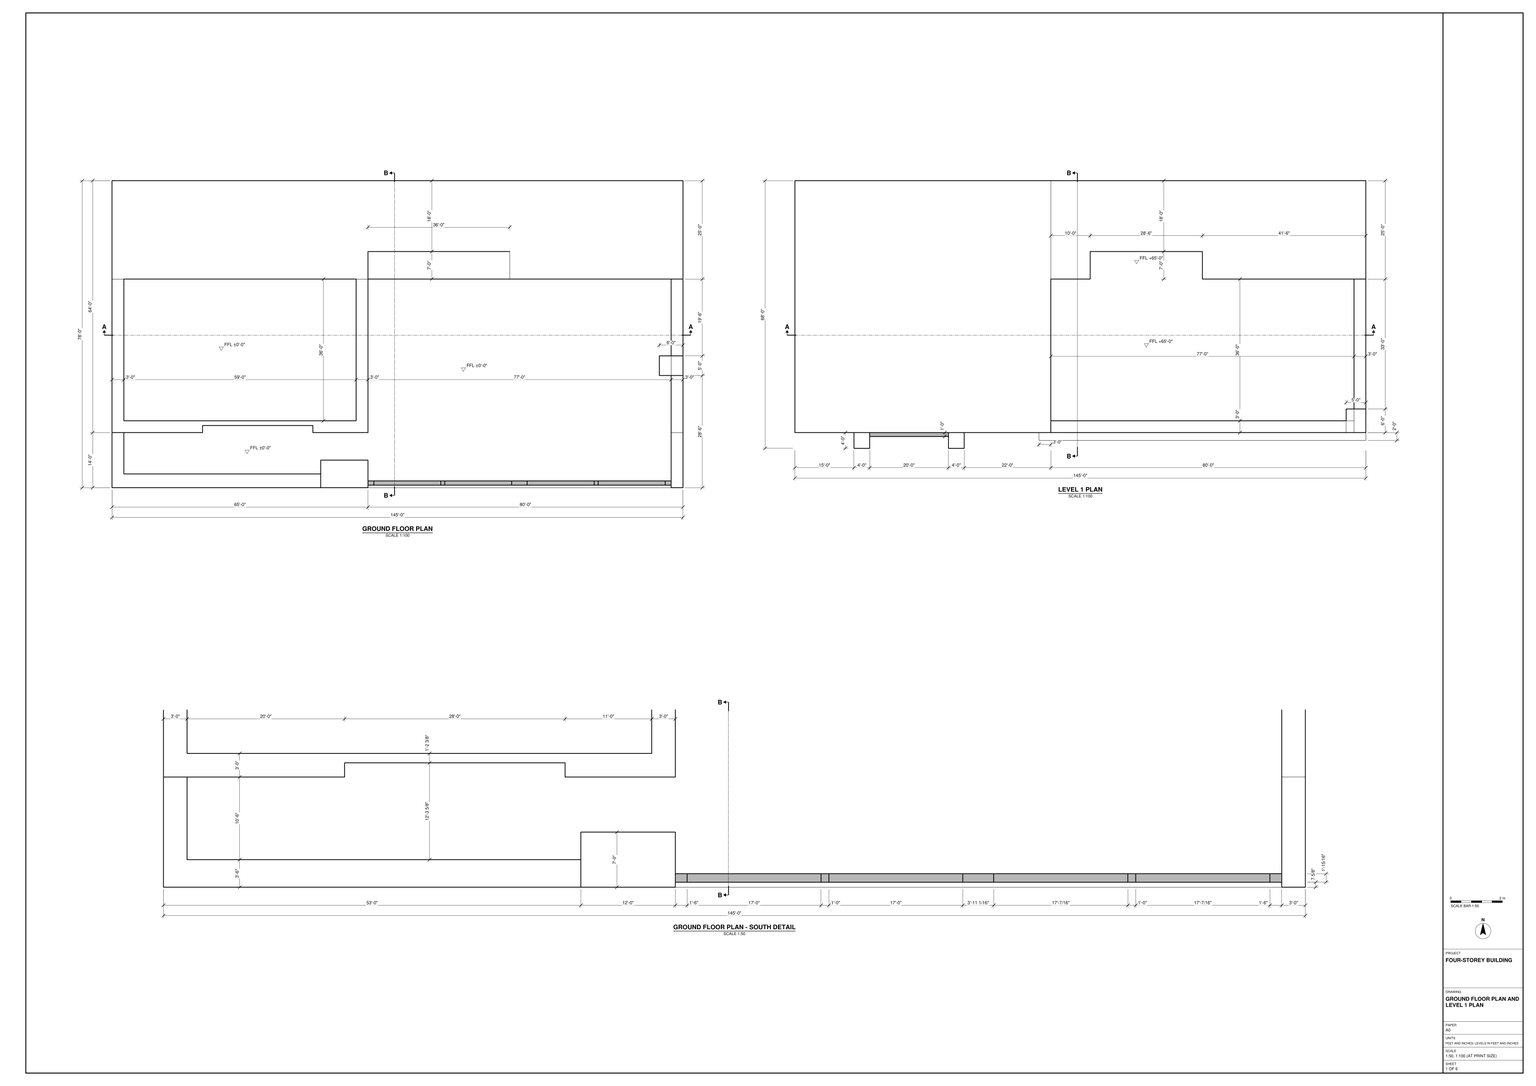
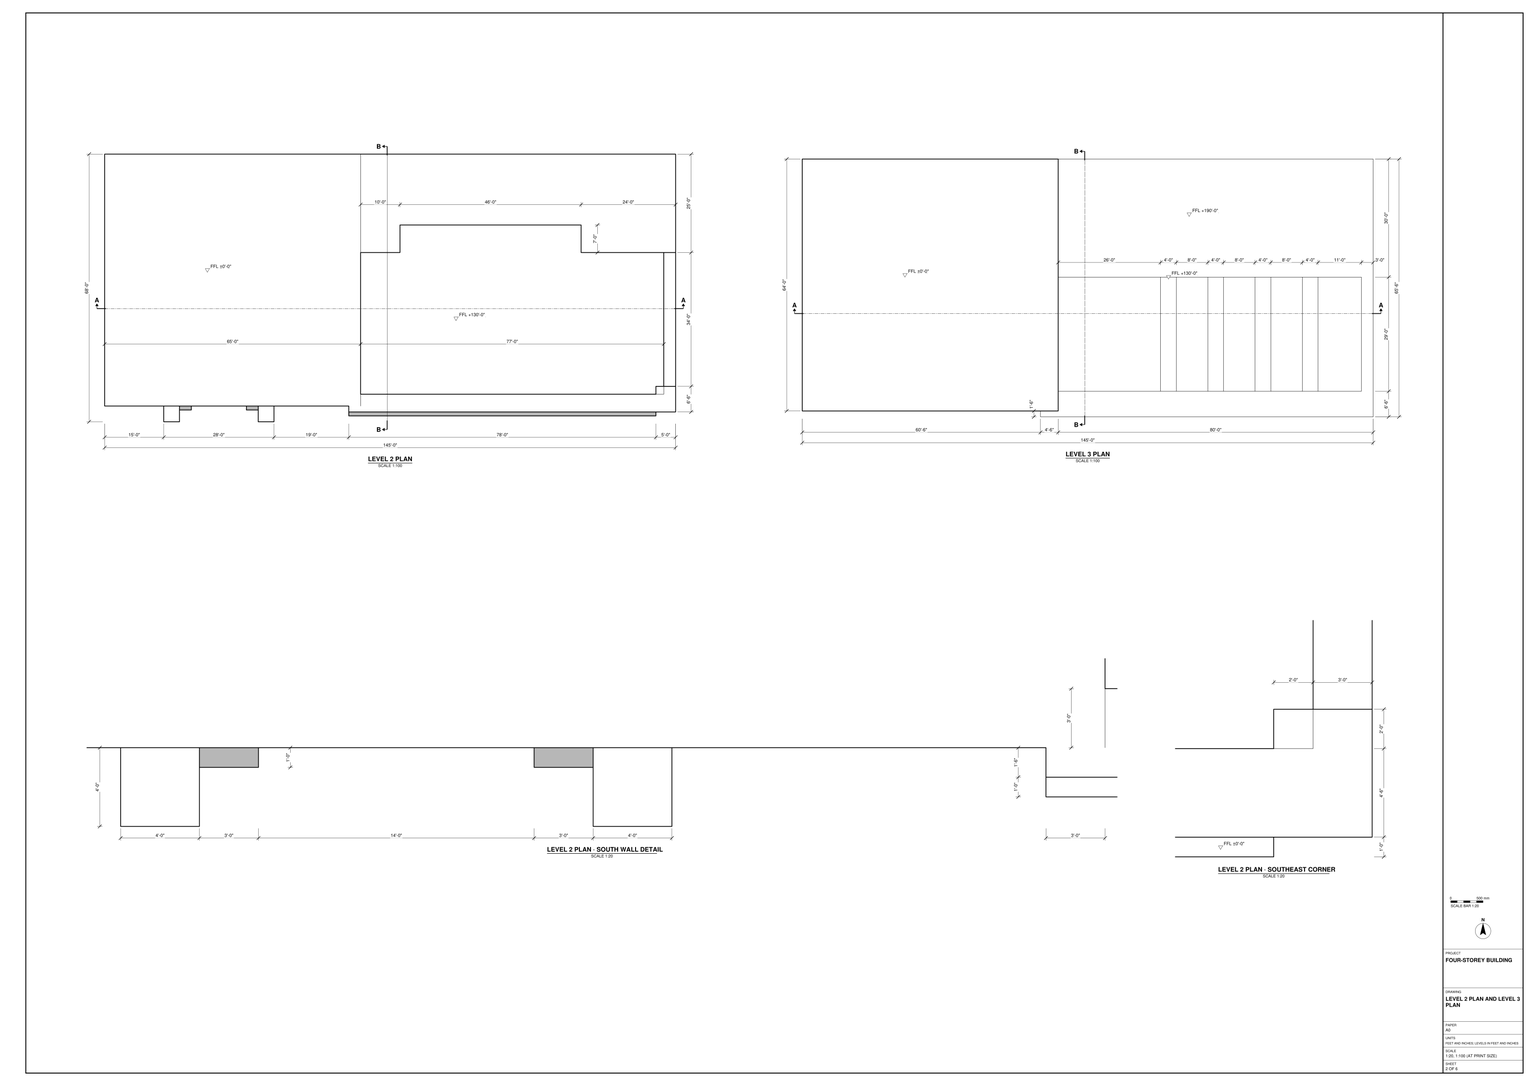
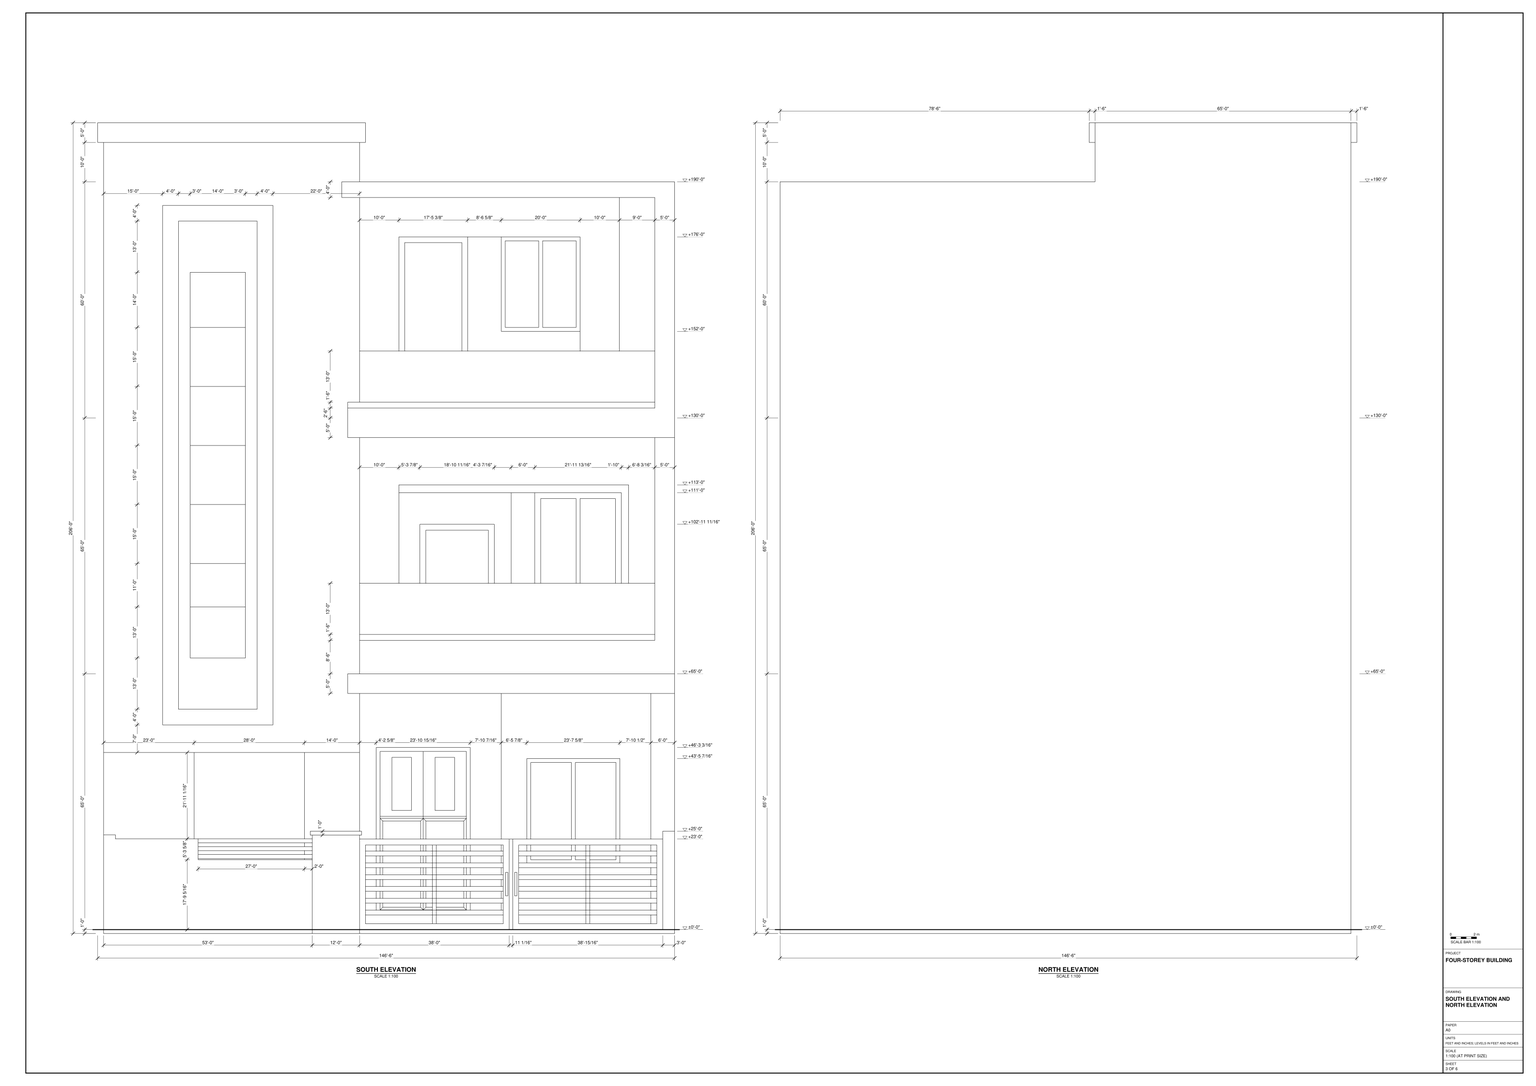
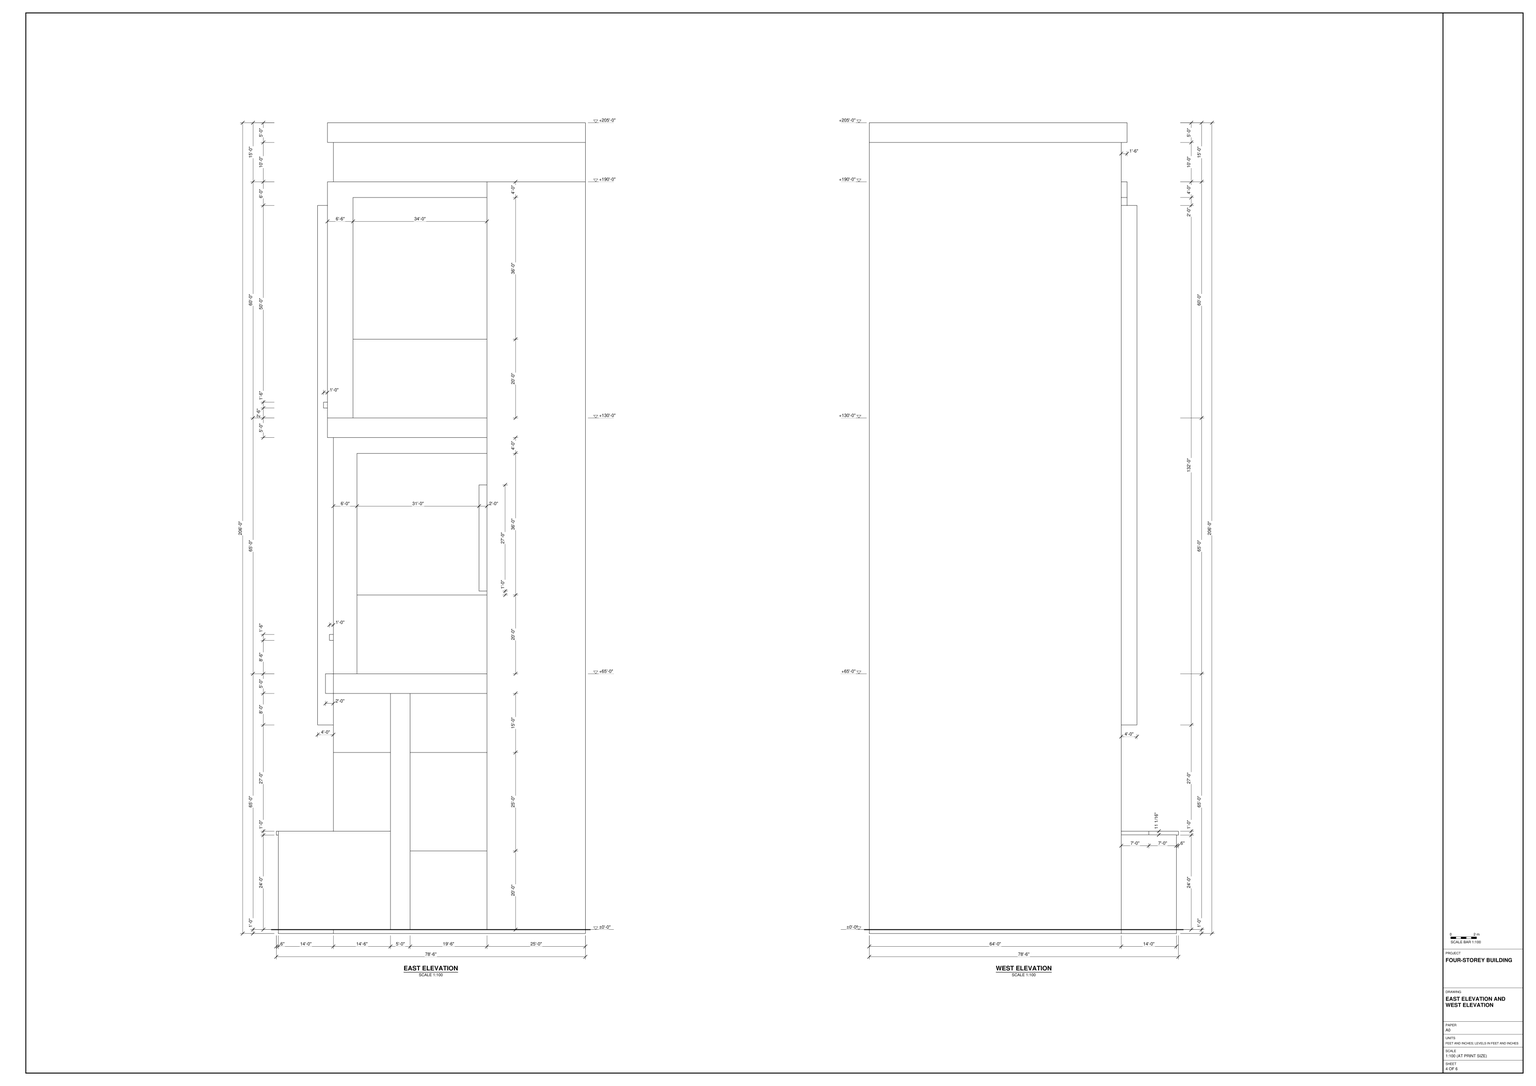
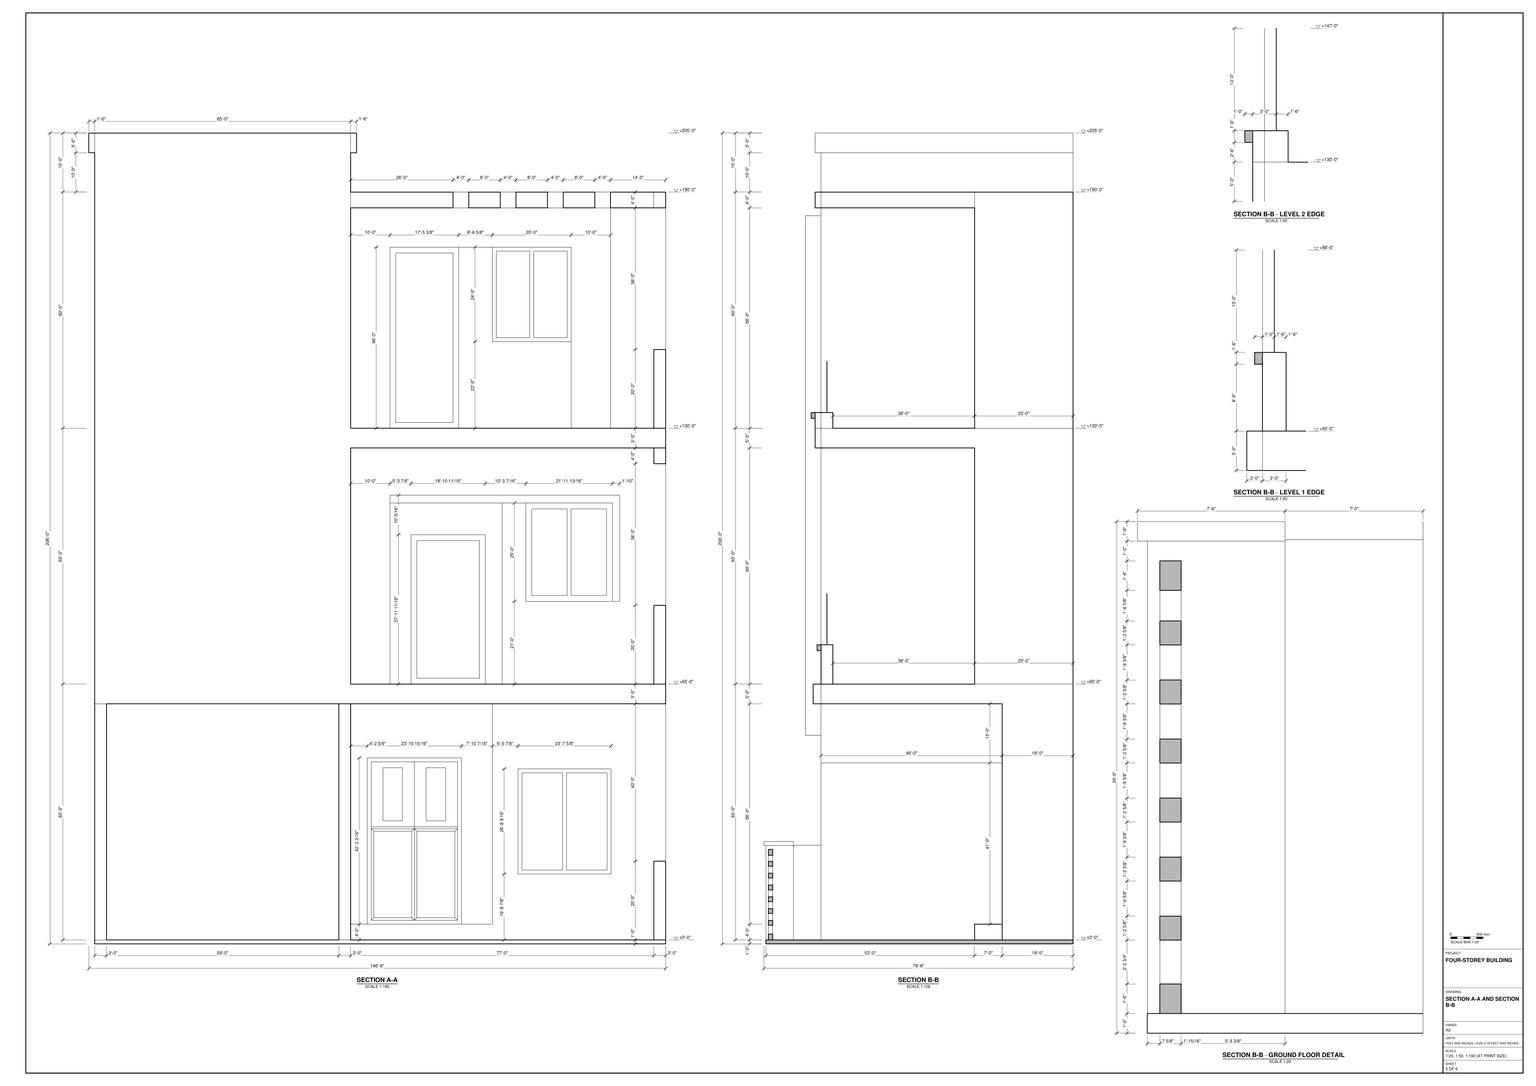
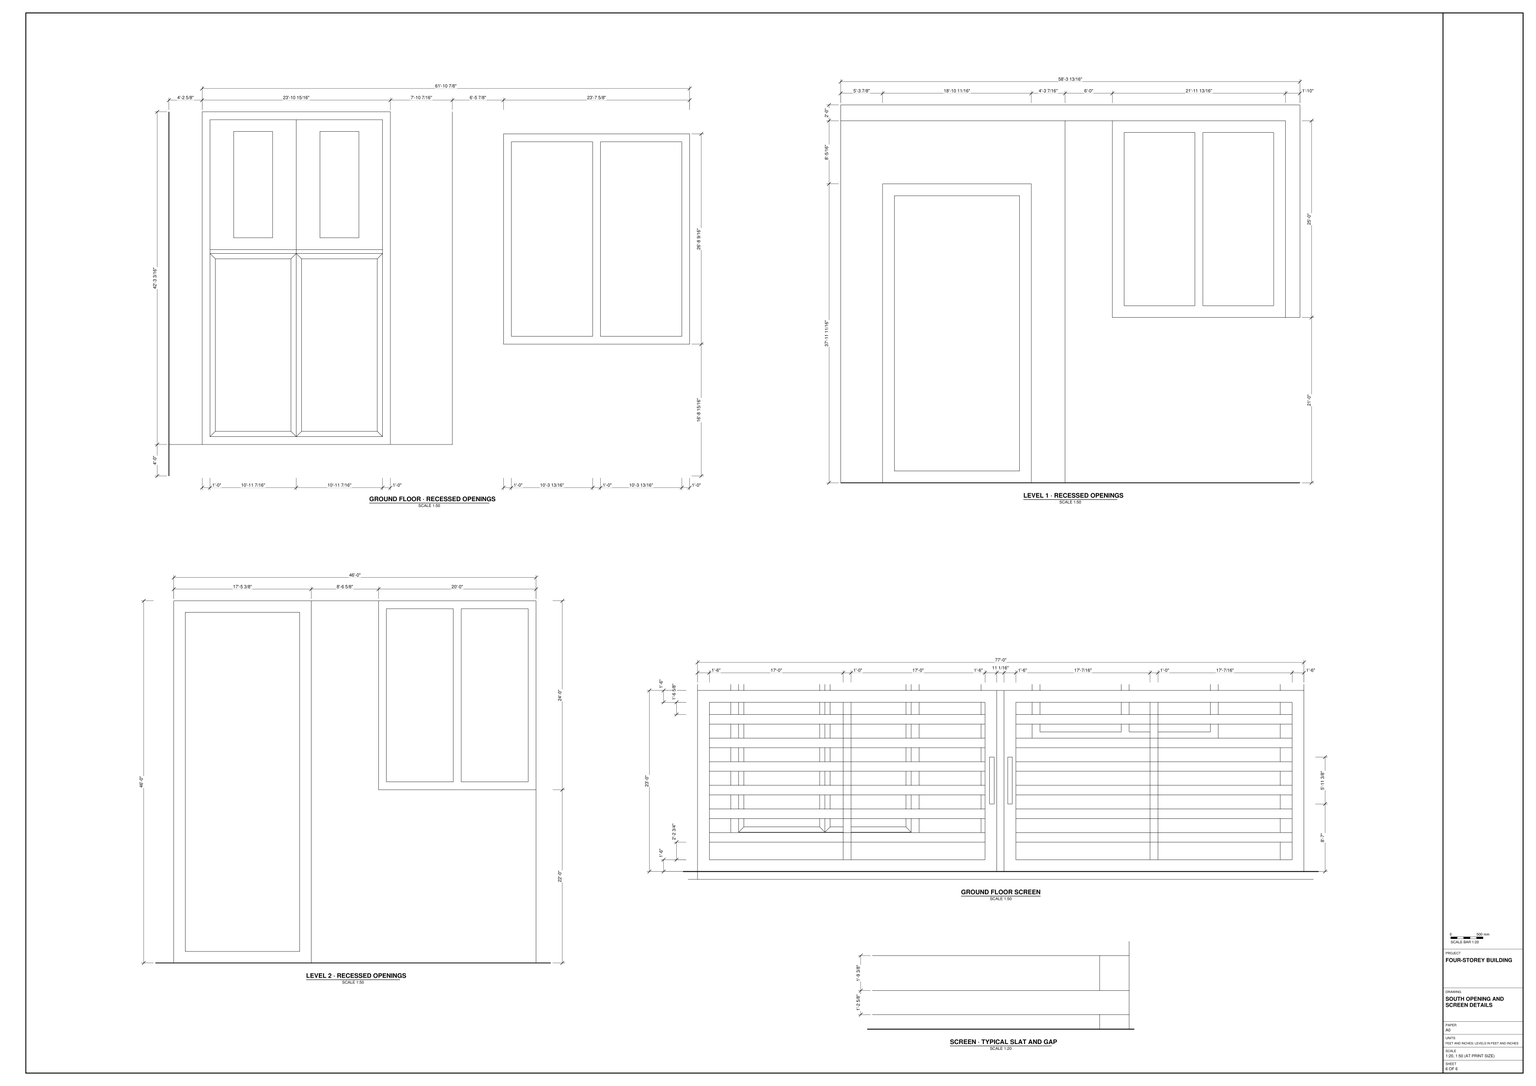
Build the four-storey building in SketchUp from task_files/diagram_01.pdf. Work in feet and inches, with the south frontage along the x-axis and the building depth along the y-axis. Including projections, the overall model shall be 146'-6" wide, 78'-6" deep and 206'-0" high. Set the floor levels at ±0'-0", +65'-0", +130'-0" and +190'-0" relative to the ground floor.

Use the plans to trace the wall returns at their drawn thicknesses and to shape the slabs and roof at each level. On the south elevation, distinguish the taller western block, with its projecting roof cap and tall framed panel, from the eastern bays. Set the upper doors and windows behind the balcony fronts so the recesses have depth. At ground level, model the frontage wall, piers and horizontally slatted gates in front of the openings. Follow the level 3 plan for the arrangement of parallel members over the eastern bays, and retain the plain stepped profile on the north elevation.

Keep shell elements such as walls, slabs and roof in separate groups or components. Keep each furniture or joinery piece shown separate as well, and use components for repeated parts. Any decor or loose items shown may use suitable library components. Save one SketchUp model as output_files/four_storey_building_with_recessed_south_balconies.skp.

# SketchUp Ruby script. Lengths in inches.
U = 1.inch
M = Sketchup.active_model
def pt(a) = Geom::Point3d.new(a.map { |v| v * U })
def face(e, loops, mat)
  f = e.add_face(loops[0].map { |a| pt(a) })
  loops[1..].each { |l| e.add_face(l.map { |a| pt(a) }).erase! }
  f.material = f.back_material = mat if mat
  f
end
# faces: each face lists its corners as indices into pts; further lists are holes
def faces(e, pts, list, mat = nil) = list.each { |f| face(e, (f[0].is_a?(Array) ? f : [f]).map { |l| l.map { |i| pts[i] } }, mat) }
# xy, xz, yz: faces in a plane at the given z, y or x. An outline is a flat list of corners, or four numbers for a rectangle; further outlines are holes
def ring(l) = l.size == 4 ? [[l[0], l[1]], [l[2], l[1]], [l[2], l[3]], [l[0], l[3]]] : l.each_slice(2).to_a
def flat(e, list, mat, &to3) = list.each { |f| face(e, (f[0].is_a?(Array) ? f : [f]).map { |l| ring(l).map { |u, v| to3.(u, v) } }, mat) }
def xy(e, z, list, mat = nil) = flat(e, list, mat) { |x, y| [x, y, z] }
def xz(e, y, list, mat = nil) = flat(e, list, mat) { |x, z| [x, y, z] }
def yz(e, x, list, mat = nil) = flat(e, list, mat) { |y, z| [x, y, z] }
def lines(e, pts, list) = list.each { |a, b| e.add_line(pt(pts[a]), pt(pts[b])) }
# prism: a flat outline (further loops are holes) pulled along v
def prism(e, loops, v, mat = nil)
  f = face(e, loops, mat); d = Geom::Vector3d.new(v.map { |x| x * U })
  f.pushpull(f.normal.samedirection?(d) ? d.length : -d.length)
end
def box(e, o, s, mat = nil) = prism(e, [[o, [o[0] + s[0], o[1], o[2]], [o[0] + s[0], o[1] + s[1], o[2]], [o[0], o[1] + s[1], o[2]]]], [0, 0, s[2]], mat)
def at(x, y, z, deg = 0) = Geom::Transformation.translation(pt([x, y, z])) * Geom::Transformation.rotation(ORIGIN, Z_AXIS, deg.degrees)
def axes(o, x, y, z) = Geom::Transformation.new([*x, 0, *y, 0, *z, 0, *pt(o).to_a, 1])
def part(name) = M.definitions.add(name)
# library, detail: a bought-in or finely detailed component or shape, given as its bounding box
def library(name, o, s) = part(name).tap { |d| box(d.entities, o, s) }
def detail(e, o, s) = box(e.add_group.entities, o, s)
def put(e, d, t, mat = nil) = e.add_instance(d, t).tap { |i| i.material = mat if mat }
def group(e, t, mat = nil) = e.add_group.tap { |g| g.transformation = t; g.material = mat if mat }.entities
root = M.entities
M.materials.add("[0022_Maroon]").color = [71, 0, 0]
M.materials.add("[0033_NavajoWhite]").color = [255, 222, 173]
M.materials.add("[0057_DarkKhaki]").color = [189, 183, 107]
M.materials.add("[0060_GrassGreen]").color = [62, 91, 5]
M.materials.add("[0061_OliveDrab]").color = [113, 150, 37]
M.materials.add("[Cladding Siding White]").color = [168, 161, 129]
M.materials.add("[Granite Dark Gray]").color = [69, 68, 68]
M.materials.add("[Stone Marble]").color = [143, 138, 136]
M.materials.add("[Translucent Glass Gray]").color = [204, 221, 91]
M.materials["[Translucent Glass Gray]"].alpha = 0.5
M.materials.add("[Translucent Glass Gray]1").color = [128, 128, 128]
M.materials["[Translucent Glass Gray]1"].alpha = 0.5
M.materials.add("[Wood Bamboo]").color = [150, 89, 36]
M.materials.add("[Wood Cherry Original]").color = [152, 86, 42]
M.materials.add("[Wood Veneer 01]").color = [120, 70, 37]
xy(root,0,[[18,6,18,174,294,174,294,195.6,630,195.6,630,6],[630,6,1758,174],[18,174,18,942,1758,942,1758,174,630,174,630,195.6,294,195.6,294,174]])
xy(root,12,[[18,6,18,174,54,174,54,48,654,48,654,6],[798,6,1722,13.64],[1722,6,1758,174],[798,13.64,1722,26.59],[1722,174,1758,348],
  [54,210,762,642],[1686,348,1722,408],[1722,348,1758,408],[1722,408,1758,642],[18,642,18,942,1758,942,1758,642,1230,642,1230,726,798,726,798,642],
  [798,642,1230,726]])
xy(root,12,[[798,26.59,1722,26.59,1722,348,1686,348,1686,408,1722,408,1722,642,798,642,798,174,630,174,630,195.6,294,195.6,294,174,54,174,54,48,654,48,654,90,798,90]],"[Granite Dark Gray]")
xy(root,30,[[816,13.64,1020,26.59],[1032,13.64,1236,26.59],[1283.08,13.64,1487.54,26.59],[1499.54,13.64,1704,26.59]])
xy(root,56.76,[[816,13.64,1236,26.59],[1283.08,13.64,1704,26.59]])
xy(root,60,[[798,642,1230,726]],"[0057_DarkKhaki]")
xy(root,71.36,[[816,13.64,1236,26.59],[1283.08,13.64,1704,26.59]])
xy(root,92.76,[[816,13.64,1236,26.59],[1283.08,13.64,1704,26.59]])
xy(root,107.36,[[816,13.64,1236,26.59],[1283.08,13.64,1704,26.59]])
xy(root,128.76,[[816,13.64,1236,26.59],[1283.08,13.64,1704,26.59]])
xy(root,143.36,[[816,13.64,1236,26.59],[1283.08,13.64,1704,26.59]])
xy(root,164.76,[[816,13.64,1236,26.59],[1283.08,13.64,1704,26.59]])
xy(root,179.36,[[816,13.64,1236,26.59],[1283.08,13.64,1704,26.59]])
xy(root,200.76,[[816,13.64,1236,26.59],[1283.08,13.64,1704,26.59]])
xy(root,215.36,[[816,13.64,1236,26.59],[1283.08,13.64,1704,26.59]])
xy(root,225.34,[[306,6,654,48]],"[0033_NavajoWhite]")
xy(root,228.5,[[306,16.5,654,38.4375]])
xy(root,236.76,[[816,13.64,1236,26.59],[1283.08,13.64,1704,26.59]])
xy(root,240.9375,[[306,16.5,654,38.4375]])
xy(root,251.36,[[816,13.64,1236,26.59],[1283.08,13.64,1704,26.59]])
xy(root,252,[[1722,408,1758,642]],"[0033_NavajoWhite]")
xy(root,252.5,[[306,16.5,654,38.4375]])
xy(root,264.9375,[[306,16.5,654,38.4375]])
xy(root,270,[[816,13.64,1020,26.59],[1032,13.64,1236,26.59],[1283.08,13.64,1487.54,26.59],[1499.54,13.64,1704,26.59]])
xy(root,276.5,[[306,16.5,654,38.4375]])
xy(root,288,[[798,13.64,1722,26.59]])
xy(root,288.9375,[[306,16.5,654,38.4375]])
xy(root,288.9375,[[54,6,306,48]],"[0033_NavajoWhite]")
xy(root,300,[[648,0,654,6],[654,0,654,6,798,6,798,90,804,90,804,0],[648,6,654,90]])
xy(root,300.9375,[[18,6,54,174]],"[0033_NavajoWhite]")
xy(root,312,[[648,0,804,90]])
xy(root,312,[[1722,6,1758,348]],"[0033_NavajoWhite]")
xy(root,552,[[294,174,630,195.6]],"[0061_OliveDrab]")
xy(root,636,[[198,126,534,174]])
xy(root,684,[[246,126,486,162],[246,162,486,174]])
xy(root,732,[[762,174,798,642],[54,210,762,642],[862.31,212.47,857.66,213.09,853.31,214.89,849.59,217.75,846.73,221.47,844.93,225.82,844.31,230.47,844.93,235.13,846.73,239.47,849.59,243.2,853.31,246.0625,857.66,247.86,862.31,248.47,866.97,247.86,871.31,246.0625,875.04,243.2,877.9,239.47,879.7,235.13,880.31,230.47,879.7,225.82,877.9,221.47,875.04,217.75,871.31,214.89,866.97,213.09],[1042.31,212.47,1037.66,213.09,1033.31,214.89,1029.59,217.75,1026.73,221.47,1024.93,225.82,1024.31,230.47,1024.93,235.13,1026.73,239.47,1029.59,243.2,1033.31,246.0625,1037.66,247.86,1042.31,248.47,1046.97,247.86,1051.31,246.0625,1055.04,243.2,1057.9,239.47,1059.7,235.13,1060.31,230.47,1059.7,225.82,1057.9,221.47,1055.04,217.75,1051.31,214.89,1046.97,213.09],[1222.31,212.47,1217.66,213.09,1213.31,214.89,1209.59,217.75,1206.73,221.47,1204.93,225.82,1204.31,230.47,1204.93,235.13,1206.73,239.47,1209.59,243.2,1213.31,246.0625,1217.66,247.86,1222.31,248.47,1226.97,247.86,1231.31,246.0625,1235.04,243.2,1237.9,239.47,1239.7,235.13,1240.31,230.47,1239.7,225.82,1237.9,221.47,1235.04,217.75,1231.31,214.89,1226.97,213.09],
  [1402.31,212.47,1397.66,213.09,1393.31,214.89,1389.59,217.75,1386.73,221.47,1384.93,225.82,1384.31,230.47,1384.93,235.13,1386.73,239.47,1389.59,243.2,1393.31,246.0625,1397.66,247.86,1402.31,248.47,1406.97,247.86,1411.31,246.0625,1415.04,243.2,1417.9,239.47,1419.7,235.13,1420.31,230.47,1419.7,225.82,1417.9,221.47,1415.04,217.75,1411.31,214.89,1406.97,213.09],[1582.31,212.47,1577.66,213.09,1573.31,214.89,1569.59,217.75,1566.73,221.47,1564.93,225.82,1564.31,230.47,1564.93,235.13,1566.73,239.47,1569.59,243.2,1573.31,246.0625,1577.66,247.86,1582.31,248.47,1586.97,247.86,1591.31,246.0625,1595.04,243.2,1597.9,239.47,1599.7,235.13,1600.31,230.47,1599.7,225.82,1597.9,221.47,1595.04,217.75,1591.31,214.89,1586.97,213.09],[1686,348,1758,408]])
xy(root,732,[[[762,150,762,174,798,174,798,726,1230,726,1230,642,1758,642,1758,408,1686,408,1686,348,1758,348,1758,150],[862.31,212.47,866.97,213.09,871.31,214.89,875.04,217.75,877.9,221.47,879.7,225.82,880.31,230.47,879.7,235.13,877.9,239.47,875.04,243.2,871.31,246.0625,866.97,247.86,862.31,248.47,857.66,247.86,853.31,246.0625,849.59,243.2,846.73,239.47,844.93,235.13,844.31,230.47,844.93,225.82,846.73,221.47,849.59,217.75,853.31,214.89,857.66,213.09],[1042.31,212.47,1046.97,213.09,1051.31,214.89,1055.04,217.75,1057.9,221.47,1059.7,225.82,1060.31,230.47,1059.7,235.13,1057.9,239.47,1055.04,243.2,1051.31,246.0625,1046.97,247.86,1042.31,248.47,1037.66,247.86,1033.31,246.0625,1029.59,243.2,1026.73,239.47,1024.93,235.13,1024.31,230.47,1024.93,225.82,1026.73,221.47,1029.59,217.75,1033.31,214.89,1037.66,213.09],[1222.31,212.47,1226.97,213.09,1231.31,214.89,1235.04,217.75,1237.9,221.47,1239.7,225.82,1240.31,230.47,1239.7,235.13,1237.9,239.47,1235.04,243.2,1231.31,246.0625,1226.97,247.86,1222.31,248.47,1217.66,247.86,1213.31,246.0625,1209.59,243.2,1206.73,239.47,1204.93,235.13,1204.31,230.47,1204.93,225.82,1206.73,221.47,1209.59,217.75,1213.31,214.89,1217.66,213.09],[1402.31,212.47,1406.97,213.09,1411.31,214.89,1415.04,217.75,1417.9,221.47,1419.7,225.82,1420.31,230.47,1419.7,235.13,1417.9,239.47,1415.04,243.2,1411.31,246.0625,1406.97,247.86,1402.31,248.47,1397.66,247.86,1393.31,246.0625,1389.59,243.2,1386.73,239.47,1384.93,235.13,1384.31,230.47,1384.93,225.82,1386.73,221.47,1389.59,217.75,1393.31,214.89,1397.66,213.09],[1582.31,212.47,1586.97,213.09,1591.31,214.89,1595.04,217.75,1597.9,221.47,1599.7,225.82,1600.31,230.47,1599.7,235.13,1597.9,239.47,1595.04,243.2,1591.31,246.0625,1586.97,247.86,1582.31,248.47,1577.66,247.86,1573.31,246.0625,1569.59,243.2,1566.73,239.47,1564.93,235.13,1564.31,230.47,1564.93,225.82,1566.73,221.47,1569.59,217.75,1573.31,214.89,1577.66,213.09]]],"[Wood Cherry Original]")
xy(root,792,[[798,174,1698,210],[1698,174,1722,210],[1722,174,1758,246],[1698,210,1722,246],[1722,246,1758,642]])
xy(root,792,[[762,150,1758,174]],"[0060_GrassGreen]")
xy(root,792,[[798,210,1698,210,1698,246,1722,246,1722,642,1260,642,1260,726,918,726,918,642,798,642]],"[Stone Marble]")
xy(root,840,[[282,162,450,174]])
xy(root,894,[[798,162,1698,174]])
xy(root,912,[[798,162,1698,174],[798,174,1698,192],[798,192,1698,210]])
xy(root,1032,[[1722,246,1758,642]],"[0033_NavajoWhite]")
xy(root,1044,[[1595.8125,618,1617.8125,642]])
xy(root,1344,[[918,618,918,726,1260,726,1260,642,1595.8125,642,1595.8125,618]],"[Wood Bamboo]")
xy(root,1368,[[918,618,1617.8125,642]])
xy(root,1464,[[1722,246,1758,642]])
xy(root,1512,[[1698,174,1722,246],[1722,174,1758,642],[964.25,258.46,958.07,259.49,952.37,262.08,947.53,266.06,943.89,271.16,941.6875,277.02,941.08,283.26,942.11,289.44,944.7,295.14,948.68,299.98,953.78,303.625,959.65,305.82,965.88,306.43,972.0625,305.4,977.77,302.8125,982.6,298.83,986.25,293.73,988.45,287.87,989.05,281.63,988.03,275.45,985.43,269.75,981.45,264.91,976.36,261.27,970.49,259.07],[1228.25,258.46,1222.07,259.49,1216.37,262.08,1211.53,266.06,1207.89,271.16,1205.6875,277.02,1205.08,283.26,1206.11,289.44,1208.7,295.14,1212.68,299.98,1217.78,303.625,1223.65,305.82,1229.88,306.43,1236.0625,305.4,1241.77,302.8125,1246.6,298.83,1250.25,293.73,1252.45,287.87,1253.05,281.63,1252.03,275.45,1249.43,269.75,1245.45,264.91,1240.36,261.27,1234.49,259.07],[1492.25,258.46,1486.07,259.49,1480.37,262.08,1475.53,266.06,1471.89,271.16,1469.6875,277.02,1469.08,283.26,1470.11,289.44,1472.7,295.14,1476.68,299.98,1481.78,303.625,1487.65,305.82,1493.88,306.43,1500.0625,305.4,1505.77,302.8125,1510.6,298.83,1514.25,293.73,1516.45,287.87,1517.05,281.63,1516.03,275.45,1513.43,269.75,1509.45,264.91,1504.36,261.27,1498.49,259.07]])
xy(root,1512,[[[762,156,762,174,798,174,798,642,1722,642,1722,246,1698,246,1698,174,1758,174,1758,156],[1228.25,258.46,1234.49,259.07,1240.36,261.27,1245.45,264.91,1249.43,269.75,1252.03,275.45,1253.05,281.63,1252.45,287.87,1250.25,293.73,1246.6,298.83,1241.77,302.8125,1236.0625,305.4,1229.88,306.43,1223.65,305.82,1217.78,303.625,1212.68,299.98,1208.7,295.14,1206.11,289.44,1205.08,283.26,1205.6875,277.02,1207.89,271.16,1211.53,266.06,1216.37,262.08,1222.07,259.49],[1492.25,258.46,1498.49,259.07,1504.36,261.27,1509.45,264.91,1513.43,269.75,1516.03,275.45,1517.05,281.63,1516.45,287.87,1514.25,293.73,1510.6,298.83,1505.77,302.8125,1500.0625,305.4,1493.88,306.43,1487.65,305.82,1481.78,303.625,1476.68,299.98,1472.7,295.14,1470.11,289.44,1469.08,283.26,1469.6875,277.02,1471.89,271.16,1475.53,266.06,1480.37,262.08,1486.07,259.49],[964.25,258.46,970.49,259.07,976.36,261.27,981.45,264.91,985.43,269.75,988.03,275.45,989.05,281.63,988.45,287.87,986.25,293.73,982.6,298.83,977.77,302.8125,972.0625,305.4,965.88,306.43,959.65,305.82,953.78,303.625,948.68,299.98,944.7,295.14,942.11,289.44,941.08,283.26,941.6875,277.02,943.89,271.16,947.53,266.06,952.37,262.08,958.07,259.49]]],"[Wood Cherry Original]")
xy(root,1572,[[1698,210,1722,234],[1722,234,1758,642]])
xy(root,1572,[[798,210,1698,210,1698,234,1722,234,1722,642,1470,642,1470,726,918,726,918,642,798,642]],"[Stone Marble]")
xy(root,1602,[[762,144,1698,156]])
xy(root,1620,[[762,144,1698,156],[762,156,1698,156,1698,192,798,192,798,174,762,174],[798,192,1698,210]])
xy(root,1812,[[1722,234,1758,642]],"[0033_NavajoWhite]")
xy(root,2016,[[282,162,450,174]])
xy(root,2124,[[918,642,1127.375,726],[1127.375,642,1470,726]],"[Wood Bamboo]")
xy(root,2172,[[246,126,486,162],[246,162,486,174]])
xy(root,2220,[[198,126,534,174]])
xy(root,2244,[[978.39,287.6,973.73,288.22,969.39,290.02,965.66,292.875,962.8,296.6,961,300.95,960.39,305.6,961,310.26,962.8,314.6,965.66,318.33,969.39,321.19,973.73,322.99,978.39,323.6,983.04,322.99,987.39,321.19,991.11,318.33,993.97,314.6,995.77,310.26,996.39,305.6,995.77,300.95,993.97,296.6,991.11,292.875,987.39,290.02,983.04,288.22],[1660.26,287.6,1655.6,288.22,1651.26,290.02,1647.53,292.875,1644.67,296.6,1642.875,300.95,1642.26,305.6,1642.875,310.26,1644.67,314.6,1647.53,318.33,1651.26,321.19,1655.6,322.99,1660.26,323.6,1664.92,322.99,1669.26,321.19,1672.99,318.33,1675.85,314.6,1677.65,310.26,1678.26,305.6,1677.65,300.95,1675.85,296.6,1672.99,292.875,1669.26,290.02,1664.92,288.22],[978.39,442.12,973.73,442.73,969.39,444.53,965.66,447.39,962.8,451.12,961,455.46,960.39,460.12,961,464.78,962.8,469.12,965.66,472.85,969.39,475.71,973.73,477.51,978.39,478.12,983.04,477.51,987.39,475.71,991.11,472.85,993.97,469.12,995.77,464.78,996.39,460.12,995.77,455.46,993.97,451.12,991.11,447.39,987.39,444.53,983.04,442.73],[1660.26,443.92,1655.6,444.53,1651.26,446.33,1647.53,449.1875,1644.67,452.92,1642.875,457.26,1642.26,461.92,1642.875,466.58,1644.67,470.92,1647.53,474.65,1651.26,477.51,1655.6,479.3,1660.26,479.92,1664.92,479.3,1669.26,477.51,1672.99,474.65,1675.85,470.92,1677.65,466.58,1678.26,461.92,1677.65,457.26,1675.85,452.92,1672.99,449.1875,1669.26,446.33,1664.92,444.53]])
xy(root,2244,[[[744,156,744,174,798,174,798,642,1758,642,1758,234,1698,234,1698,156],[1542,234,1590,582],[1398,234,1446,582],[1254,234,1302,582],[1110,234,1158,582],[978.39,442.12,983.04,442.73,987.39,444.53,991.11,447.39,993.97,451.12,995.77,455.46,996.39,460.12,995.77,464.78,993.97,469.12,991.11,472.85,987.39,475.71,983.04,477.51,978.39,478.12,973.73,477.51,969.39,475.71,965.66,472.85,962.8,469.12,961,464.78,960.39,460.12,961,455.46,962.8,451.12,965.66,447.39,969.39,444.53,973.73,442.73],[978.39,287.6,983.04,288.22,987.39,290.02,991.11,292.875,993.97,296.6,995.77,300.95,996.39,305.6,995.77,310.26,993.97,314.6,991.11,318.33,987.39,321.19,983.04,322.99,978.39,323.6,973.73,322.99,969.39,321.19,965.66,318.33,962.8,314.6,961,310.26,960.39,305.6,961,300.95,962.8,296.6,965.66,292.875,969.39,290.02,973.73,288.22],[1660.26,287.6,1664.92,288.22,1669.26,290.02,1672.99,292.875,1675.85,296.6,1677.65,300.95,1678.26,305.6,1677.65,310.26,1675.85,314.6,1672.99,318.33,1669.26,321.19,1664.92,322.99,1660.26,323.6,1655.6,322.99,1651.26,321.19,1647.53,318.33,1644.67,314.6,1642.875,310.26,1642.26,305.6,1642.875,300.95,1644.67,296.6,1647.53,292.875,1651.26,290.02,1655.6,288.22],[1660.26,443.92,1664.92,444.53,1669.26,446.33,1672.99,449.1875,1675.85,452.92,1677.65,457.26,1678.26,461.92,1677.65,466.58,1675.85,470.92,1672.99,474.65,1669.26,477.51,1664.92,479.3,1660.26,479.92,1655.6,479.3,1651.26,477.51,1647.53,474.65,1644.67,470.92,1642.875,466.58,1642.26,461.92,1642.875,457.26,1644.67,452.92,1647.53,449.1875,1651.26,446.33,1655.6,444.53]]],"[0033_NavajoWhite]")
xy(root,2292,[[744,156,1758,156,1758,942,798,942,798,582,1722,582,1722,234,798,234,798,174,744,174],[798,234,1110,582],[1158,234,1254,582],[1302,234,1398,582],[1446,234,1542,582],
  [1590,234,1722,582]],"[0057_DarkKhaki]")
xy(root,2412,[[0,156,0,942,18,942,18,174,798,174,798,942,816,942,816,156]],"[0060_GrassGreen]")
xy(root,2472,[[0,156,816,942]])
xz(root,0,[[648,300,804,312]])
xz(root,6,[[654,0,798,300],[798,0,1758,12]])
xz(root,6,[[18,0,654,12],[18,12,654,12,654,225.34,306,225.34,306,288.9375,54,288.9375,54,300.9375,18,300.9375],[1722,12,1758,312]],"[0033_NavajoWhite]")
xz(root,13.64,[[[798,12,1254,288],[816,30,1236,270],[1243,115.02,1250,186.39]],[1254,12,1265.08,288],[[1265.08,12,1722,288],[1283.08,30,1704,270],[1270.62,115.02,1277.62,186.39]],[1020,30,1032,56.76],[1487.54,30,1499.54,56.76],
  [816,56.76,1020,71.36],[1020,56.76,1032,71.36],[1032,56.76,1236,71.36],[1283.08,56.76,1487.54,71.36],[1487.54,56.76,1499.54,71.36],
  [1499.54,56.76,1704,71.36],[1020,71.36,1032,92.76],[1487.54,71.36,1499.54,92.76],[816,92.76,1020,107.36],[1020,92.76,1032,107.36],
  [1032,92.76,1236,107.36],[1283.08,92.76,1487.54,107.36],[1487.54,92.76,1499.54,107.36],[1499.54,92.76,1704,107.36],[1020,107.36,1032,128.76],
  [1487.54,107.36,1499.54,128.76],[1243,115.02,1250,186.39],[1270.62,115.02,1277.62,186.39],[816,128.76,1020,143.36],[1020,128.76,1032,143.36],
  [1032,128.76,1236,143.36],[1283.08,128.76,1487.54,143.36],[1487.54,128.76,1499.54,143.36],[1499.54,128.76,1704,143.36],[1020,143.36,1032,164.76],
  [1487.54,143.36,1499.54,164.76],[816,164.76,1020,179.36],[1020,164.76,1032,179.36],[1032,164.76,1236,179.36],[1283.08,164.76,1487.54,179.36],
  [1487.54,164.76,1499.54,179.36],[1499.54,164.76,1704,179.36],[1020,179.36,1032,200.76],[1487.54,179.36,1499.54,200.76],[816,200.76,1020,215.36],
  [1020,200.76,1032,215.36],[1032,200.76,1236,215.36],[1283.08,200.76,1487.54,215.36],[1487.54,200.76,1499.54,215.36],[1499.54,200.76,1704,215.36],
  [1020,215.36,1032,236.76],[1487.54,215.36,1499.54,236.76],[816,236.76,1020,251.36],[1020,236.76,1032,251.36],[1032,236.76,1236,251.36],
  [1283.08,236.76,1487.54,251.36],[1487.54,236.76,1499.54,251.36],[1499.54,236.76,1704,251.36],[1020,251.36,1032,270],[1487.54,251.36,1499.54,270]])
xz(root,16.5,[[306,228.5,654,240.9375],[306,252.5,654,264.9375],[306,276.5,654,288.9375]])
xz(root,26.59,[[[798,12,1722,288],[1283.08,30,1487.54,30,1487.54,56.76,1499.54,56.76,1499.54,30,1704,30,1704,270,1499.54,270,1499.54,251.36,1487.54,251.36,1487.54,270,1283.08,270],[816,30,1020,30,1020,56.76,1032,56.76,1032,30,1236,30,1236,270,1032,270,1032,251.36,1020,251.36,1020,270,816,270]],[816,56.76,1020,71.36],[1020,56.76,1032,71.36],[1032,56.76,1236,71.36],[1283.08,56.76,1487.54,71.36],
  [1487.54,56.76,1499.54,71.36],[1499.54,56.76,1704,71.36],[1020,71.36,1032,92.76],[1487.54,71.36,1499.54,92.76],[816,92.76,1020,107.36],
  [1020,92.76,1032,107.36],[1032,92.76,1236,107.36],[1283.08,92.76,1487.54,107.36],[1487.54,92.76,1499.54,107.36],[1499.54,92.76,1704,107.36],
  [1020,107.36,1032,128.76],[1487.54,107.36,1499.54,128.76],[816,128.76,1020,143.36],[1020,128.76,1032,143.36],[1032,128.76,1236,143.36],
  [1283.08,128.76,1487.54,143.36],[1487.54,128.76,1499.54,143.36],[1499.54,128.76,1704,143.36],[1020,143.36,1032,164.76],[1487.54,143.36,1499.54,164.76],
  [816,164.76,1020,179.36],[1020,164.76,1032,179.36],[1032,164.76,1236,179.36],[1283.08,164.76,1487.54,179.36],[1487.54,164.76,1499.54,179.36],
  [1499.54,164.76,1704,179.36],[1020,179.36,1032,200.76],[1487.54,179.36,1499.54,200.76],[816,200.76,1020,215.36],[1020,200.76,1032,215.36],
  [1032,200.76,1236,215.36],[1283.08,200.76,1487.54,215.36],[1487.54,200.76,1499.54,215.36],[1499.54,200.76,1704,215.36],[1020,215.36,1032,236.76],
  [1487.54,215.36,1499.54,236.76],[816,236.76,1020,251.36],[1020,236.76,1032,251.36],[1032,236.76,1236,251.36],[1283.08,236.76,1487.54,251.36],
  [1487.54,236.76,1499.54,251.36],[1499.54,236.76,1704,251.36]])
xz(root,38.4375,[[306,228.5,654,240.9375],[306,252.5,654,264.9375],[306,276.5,654,288.9375]])
xz(root,48,[[54,12,54,288.9375,306,288.9375,306,225.34,654,225.34,654,12]],"[0033_NavajoWhite]")
xz(root,90,[[654,12,798,312],[648,300,654,312],[798,300,804,312]])
xz(root,126,[[[198,636,534,2220],[246,684,486,2172]]])
xz(root,144,[[762,1602,1698,1620]])
xz(root,150,[[762,732,1758,792]],"[0060_GrassGreen]")
xz(root,156,[[762,1602,1698,1620]])
xz(root,156,[[762,1512,1758,1512,1758,2292,744,2292,744,2244,1698,2244,1698,1602,762,1602]],"[0033_NavajoWhite]")
xz(root,156,[[0,2412,816,2472]],"[0060_GrassGreen]")
xz(root,162,[[798,894,1698,912]])
xz(root,162,[[[246,684,486,2172],[282,840,450,2016]]],"[0061_OliveDrab]")
xz(root,174,[[18,0,294,12],[630,0,798,12],[18,12,54,300.9375],[[198,636,534,2220],[246,684,486,2172]],[[246,684,486,2172],[282,840,450,2016]],
  [798,894,1698,912]])
xz(root,174,[[798,792,1758,792,1758,1512,1698,1512,1698,894,798,894]],"[0033_NavajoWhite]")
xz(root,174,[[630,12,798,552]],"[0057_DarkKhaki]")
xz(root,174,[[54,12,294,12,294,552,18,552,18,300.9375,54,300.9375]],"[0060_GrassGreen]")
xz(root,174,[[[18,552,798,552,798,732,762,732,762,792,798,792,798,1512,762,1512,762,1620,798,1620,798,2244,744,2244,744,2292,798,2292,798,2412,18,2412],[198,636,534,2220]]],"[Cladding Siding White]")
xz(root,174,[[282,840,450,996],[282,996,450,1128],[282,1128,450,1308],[282,1308,450,1488],[282,1488,450,1668],
  [282,1668,450,1848],[282,1848,450,2016]],"[Translucent Glass Gray]")
xz(root,192,[[798,912,1698,1068],[798,1620,1698,1776]],"[Translucent Glass Gray]1")
xz(root,195.6,[[294,0,630,12]])
xz(root,195.6,[[294,12,630,552]],"[0061_OliveDrab]")
xz(root,210,[[54,12,762,732],[798,792,1698,912],[798,1572,1698,1620]])
xz(root,234,[[1698,1572,1698,2244,1758,2244,1758,1812,1722,1812,1722,1572],[1722,1572,1758,1812],[1110,2244,1158,2292],[1254,2244,1302,2292],[1398,2244,1446,2292],
  [1542,2244,1590,2292]])
xz(root,246,[[1698,792,1722,1032],[1722,792,1758,1032],[1698,1032,1722,1464],[1722,1032,1758,1464],[1698,1464,1722,1512]])
xz(root,348,[[1722,12,1758,312]])
xz(root,348,[[1686,12,1722,12,1722,312,1758,312,1758,732,1686,732]],"[0057_DarkKhaki]")
xz(root,408,[[1722,12,1758,252]])
xz(root,408,[[1686,12,1686,732,1758,732,1758,252,1722,252,1722,12]],"[0057_DarkKhaki]")
xz(root,582,[[1110,2244,1158,2292],[1254,2244,1302,2292],[1398,2244,1446,2292],[1542,2244,1590,2292]])
xz(root,618,[[1595.8125,1044,1617.8125,1044,1617.8125,1368,918,1368,918,1344,1595.8125,1344]])
xz(root,642,[[54,12,762,732],[1722,12,1758,252],[1722,792,1758,1032],[1722,1464,1758,1512],[1722,1572,1758,1812]])
xz(root,642,[[[1307.9,212.89,1591.53,533.45],[1455.71,224.89,1579.53,521.45],[1319.9,224.89,1443.71,521.45]],[[1332,1044,1595.8125,1344],[1469.91,1062,1577.8125,1326],[1350,1062,1457.91,1326]]],"[0022_Maroon]")
xz(root,642,[[[798,12,1722,12,1722,252,1758,252,1758,732,1230,732,1230,60,798,60],[1307.9,212.89,1591.53,533.45]],[798,1572,918,1572,918,2124,1470,2124,1470,1572,1590,1572,1590,2244,798,2244]],"[0057_DarkKhaki]")
xz(root,642,[[798,792,918,792,918,1368,1617.8125,1368,1617.8125,1044,1332,1044,1332,1344,1260,1344,1260,792,1722,792,1722,1032,1758,1032,1758,1464,1722,1464,1722,1512,798,1512],[1590,1572,1722,1572,1722,1812,1758,1812,1758,2244,1590,2244]],"[0061_OliveDrab]")
xz(root,642,[[1319.9,224.89,1443.71,521.45],[1455.71,224.89,1579.53,521.45],[1350,1062,1457.91,1326],[1469.91,1062,1577.8125,1326]],"[Translucent Glass Gray]")
xz(root,726,[[798,12,1230,60]])
xz(root,726,[[[1230,1836,1470,2124],[1356,1848,1458,2112],[1242,1848,1344,2112]]],"[0022_Maroon]")
xz(root,726,[[1127.375,1572,1470,1572,1470,1836,1230,1836,1230,2124,1127.375,2124]],"[0061_OliveDrab]")
xz(root,726,[[1242,1848,1344,2112],[1356,1848,1458,2112]],"[Translucent Glass Gray]")
xz(root,726,[[896.64,375.1875,956.1,537.1875],[1028.1,375.1875,1087.57,537.1875]],"[Translucent Glass Gray]1")
xz(root,726,[[798,60,848.64,60,848.64,567.1875,1135.57,567.1875,1135.57,60,1230,60,1230,732,798,732],[918,792,981.88,792,981.88,1247.6875,1208.57,1247.6875,1208.57,792,1260,792,1260,1344,918,1344]],"[Wood Bamboo]")
xz(root,726,[[[848.64,60,1135.57,567.1875],[860.64,72,1123.57,555.1875]],[860.64,72,868.64,80,868.64,343.1875,860.64,351.1875],[860.64,72,992.1,72,984.1,80,868.64,80],[992.1,72,992.1,351.1875,984.1,343.1875,984.1,80],[992.1,72,1000.1,80,1000.1,343.1875,992.1,351.1875],
  [992.1,72,1123.57,72,1115.57,80,1000.1,80],[1123.57,72,1123.57,351.1875,1115.57,343.1875,1115.57,80],[868.64,80,984.1,343.1875],[1000.1,80,1115.57,343.1875],[868.64,343.1875,984.1,343.1875,992.1,351.1875,860.64,351.1875],
  [1000.1,343.1875,1115.57,343.1875,1123.57,351.1875,992.1,351.1875],[860.64,351.1875,992.1,357.1875],[992.1,351.1875,1123.57,357.1875],[[860.64,357.1875,992.1,555.1875],[896.64,375.1875,956.1,537.1875]],[[992.1,357.1875,1123.57,555.1875],[1028.1,375.1875,1087.57,537.1875]],
  [[981.88,792,1208.57,1247.6875],[999.88,810,1190.57,1229.6875]],[999.88,810,1190.57,1229.6875],[[918,1572,1127.375,2124],[935.47,1589.47,1109.91,2106.53]],[935.47,1589.47,1109.91,2106.53]],"[Wood Veneer 01]")
xz(root,942,[[18,0,1758,12],[0,2412,18,2472]])
xz(root,942,[[18,12,18,2472,798,2472,798,2292,1758,2292,1758,12]],"[0057_DarkKhaki]")
xz(root,942,[[798,2412,816,2472]],"[0060_GrassGreen]")
yz(root,0,[[156,2412,942,2472]],"[0060_GrassGreen]")
yz(root,18,[[6,0,174,12],[174,0,942,12],[6,12,174,300.9375]])
yz(root,18,[[174,12,942,2412]],"[0057_DarkKhaki]")
yz(root,54,[[210,12,642,732]])
yz(root,54,[[48,12,174,12,174,300.9375,6,300.9375,6,288.9375,48,288.9375]],"[0033_NavajoWhite]")
yz(root,198,[[126,636,174,2220]])
yz(root,246,[[126,684,162,2172],[162,684,174,2172]])
yz(root,282,[[162,840,174,2016]])
yz(root,294,[[174,0,195.6,12]])
yz(root,294,[[174,12,195.6,552]],"[0061_OliveDrab]")
yz(root,306,[[16.5,228.5,38.4375,240.9375],[16.5,252.5,38.4375,264.9375],[16.5,276.5,38.4375,288.9375]])
yz(root,306,[[[6,225.34,48,225.34,48,288.9375,38.4375,288.9375,38.4375,276.5,16.5,276.5,16.5,288.9375,6,288.9375],[16.5,252.5,38.4375,264.9375],[16.5,228.5,38.4375,240.9375]]],"[0033_NavajoWhite]")
yz(root,450,[[162,840,174,2016]])
yz(root,486,[[126,684,162,2172],[162,684,174,2172]])
yz(root,534,[[126,636,174,2220]])
yz(root,630,[[174,0,195.6,12]])
yz(root,630,[[174,12,195.6,552]],"[0061_OliveDrab]")
yz(root,648,[[0,300,90,312]])
yz(root,654,[[6,12,48,225.34],[[48,12,48,225.34,6,225.34,6,300,90,300,90,12],[16.5,252.5,38.4375,264.9375],[16.5,228.5,38.4375,240.9375],[16.5,276.5,38.4375,288.9375]]])
yz(root,744,[[156,2244,174,2292]])
yz(root,762,[[210,12,642,732],[156,1512,174,1572],[156,1572,174,1620],[144,1602,156,1620]])
yz(root,762,[[150,732,174,792]],"[0060_GrassGreen]")
yz(root,798,[[6,12,13.64,12,13.64,288,26.59,288,26.59,12,90,12,90,300,6,300],[13.64,12,26.59,288],[642,12,726,60],[174,792,210,912],[162,894,174,912]])
yz(root,798,[[174,12,642,12,642,60,726,60,726,552,174,552],[174,552,726,732],[210,792,642,792,642,1512,174,1512,174,912,210,912],[210,1572,642,1572,642,2244,174,2244,174,1620,210,1620],[174,2292,942,2412]],"[0057_DarkKhaki]")
yz(root,804,[[0,300,90,312]])
yz(root,816,[[13.64,30,26.59,56.76],[13.64,56.76,26.59,71.36],[13.64,71.36,26.59,92.76],[13.64,92.76,26.59,107.36],[13.64,107.36,26.59,128.76],
  [13.64,128.76,26.59,143.36],[13.64,143.36,26.59,164.76],[13.64,164.76,26.59,179.36],[13.64,179.36,26.59,200.76],[13.64,200.76,26.59,215.36],
  [13.64,215.36,26.59,236.76],[13.64,236.76,26.59,251.36],[13.64,251.36,26.59,270]])
yz(root,816,[[156,2412,942,2472]],"[0060_GrassGreen]")
yz(root,918,[[618,1344,642,1368]])
yz(root,918,[[642,792,726,1344],[642,1572,726,2124]],"[Wood Bamboo]")
yz(root,1020,[[13.64,30,26.59,270]])
yz(root,1032,[[13.64,30,26.59,270]])
yz(root,1110,[[234,2244,582,2292]])
yz(root,1158,[[234,2244,582,2292]])
yz(root,1230,[[642,60,726,732]],"[Wood Bamboo]")
yz(root,1236,[[13.64,30,26.59,56.76],[13.64,56.76,26.59,71.36],[13.64,71.36,26.59,92.76],[13.64,92.76,26.59,107.36],[13.64,107.36,26.59,128.76],
  [13.64,128.76,26.59,143.36],[13.64,143.36,26.59,164.76],[13.64,164.76,26.59,179.36],[13.64,179.36,26.59,200.76],[13.64,200.76,26.59,215.36],
  [13.64,215.36,26.59,236.76],[13.64,236.76,26.59,251.36],[13.64,251.36,26.59,270]])
yz(root,1254,[[234,2244,582,2292]])
yz(root,1260,[[642,792,726,1344]],"[Wood Bamboo]")
yz(root,1283.08,[[13.64,30,26.59,56.76],[13.64,56.76,26.59,71.36],[13.64,71.36,26.59,92.76],[13.64,92.76,26.59,107.36],[13.64,107.36,26.59,128.76],
  [13.64,128.76,26.59,143.36],[13.64,143.36,26.59,164.76],[13.64,164.76,26.59,179.36],[13.64,179.36,26.59,200.76],[13.64,200.76,26.59,215.36],
  [13.64,215.36,26.59,236.76],[13.64,236.76,26.59,251.36],[13.64,251.36,26.59,270]])
yz(root,1302,[[234,2244,582,2292]])
yz(root,1398,[[234,2244,582,2292]])
yz(root,1446,[[234,2244,582,2292]])
yz(root,1470,[[642,1572,726,2124]],"[Wood Bamboo]")
yz(root,1487.54,[[13.64,30,26.59,270]])
yz(root,1499.54,[[13.64,30,26.59,270]])
yz(root,1542,[[234,2244,582,2292]])
yz(root,1590,[[234,2244,582,2292]])
yz(root,1595.8125,[[618,1044,642,1344]])
yz(root,1617.8125,[[618,1044,642,1368]])
yz(root,1686,[[348,12,408,732]],"[0057_DarkKhaki]")
yz(root,1698,[[162,894,174,912],[144,1602,156,1620]])
yz(root,1698,[[210,792,210,912,174,912,174,1512,246,1512,246,792],[210,1572,210,1620,156,1620,156,2244,234,2244,234,1572]],"[0033_NavajoWhite]")
yz(root,1704,[[13.64,30,26.59,56.76],[13.64,56.76,26.59,71.36],[13.64,71.36,26.59,92.76],[13.64,92.76,26.59,107.36],[13.64,107.36,26.59,128.76],
  [13.64,128.76,26.59,143.36],[13.64,143.36,26.59,164.76],[13.64,164.76,26.59,179.36],[13.64,179.36,26.59,200.76],[13.64,200.76,26.59,215.36],
  [13.64,215.36,26.59,236.76],[13.64,236.76,26.59,251.36],[13.64,251.36,26.59,270]])
yz(root,1722,[[13.64,12,26.59,288],[246,1464,642,1512]])
yz(root,1722,[[6,12,6,312,348,312,348,12,26.59,12,26.59,288,13.64,288,13.64,12],[408,12,642,252],[246,792,642,1032],[234,1572,642,1812]],"[0033_NavajoWhite]")
yz(root,1758,[[6,0,174,12],[174,0,942,12]])
yz(root,1758,[[6,12,348,312],[408,12,642,252],[174,732,642,792],[174,792,246,792,246,1464,642,1464,642,1512,174,1512],[246,792,642,1032],
  [156,1512,642,1572],[156,1572,234,1572,234,2244,642,2244,642,2292,156,2292],[234,1572,642,1812]],"[0033_NavajoWhite]")
yz(root,1758,[[348,12,408,732],[642,12,942,2292]],"[0057_DarkKhaki]")
yz(root,1758,[[150,732,174,792]],"[0060_GrassGreen]")
p = [[54,642,732],[18,642,732],[54,174,732],[54,210,732],[798,642,792],[798,942,792],
  [798,174,1572],[798,210,1572],[798,642,1572],[798,942,1572],[1722,642,2292],[1722,642,2244],
  [798,642,2244],[798,642,2292]]
lines(root,p,[[0,1],[2,3],[4,5],[6,7],[8,9],[10,11],[12,13]])
